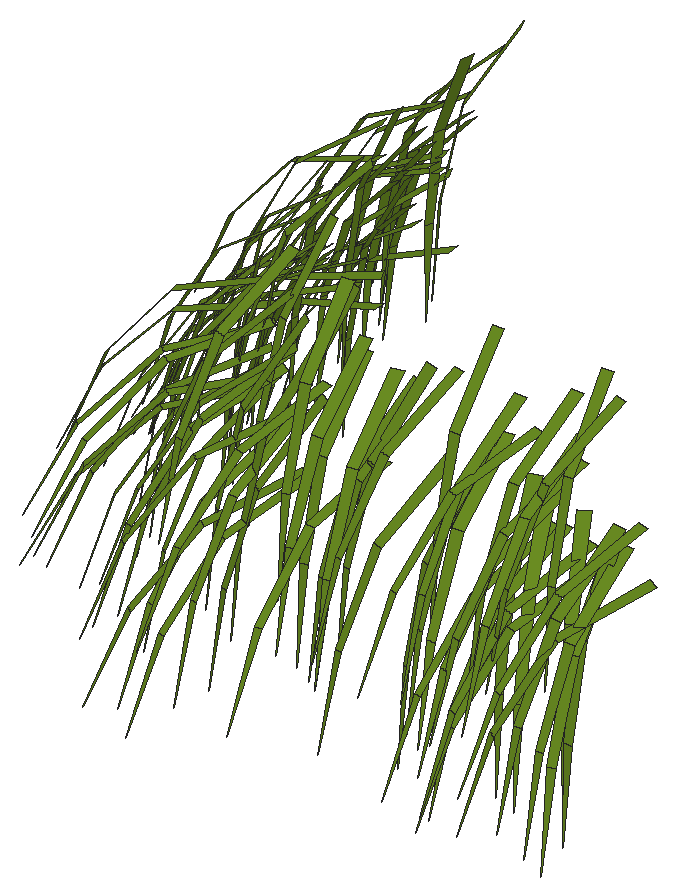
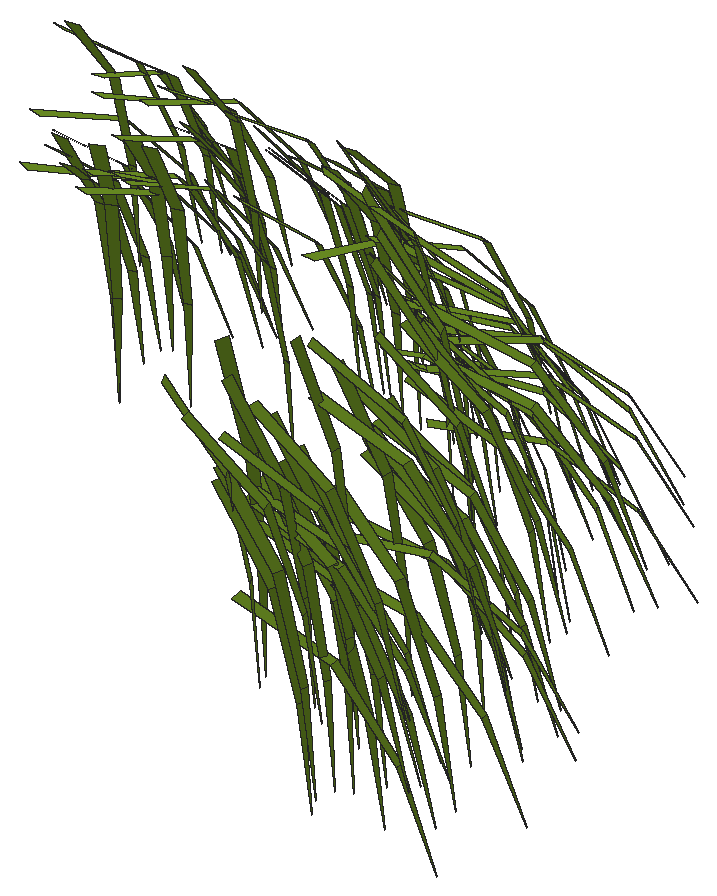
# SketchUp Ruby script. Lengths in inches.
U = 1.inch
M = Sketchup.active_model
def pt(a) = Geom::Point3d.new(a.map { |v| v * U })
def face(e, loops, mat)
  f = e.add_face(loops[0].map { |a| pt(a) })
  loops[1..].each { |l| e.add_face(l.map { |a| pt(a) }).erase! }
  f.material = f.back_material = mat if mat
  f
end
# faces: each face lists its corners as indices into pts; further lists are holes
def faces(e, pts, list, mat = nil) = list.each { |f| face(e, (f[0].is_a?(Array) ? f : [f]).map { |l| l.map { |i| pts[i] } }, mat) }
# xy, xz, yz: faces in a plane at the given z, y or x. An outline is a flat list of corners, or four numbers for a rectangle; further outlines are holes
def ring(l) = l.size == 4 ? [[l[0], l[1]], [l[2], l[1]], [l[2], l[3]], [l[0], l[3]]] : l.each_slice(2).to_a
def flat(e, list, mat, &to3) = list.each { |f| face(e, (f[0].is_a?(Array) ? f : [f]).map { |l| ring(l).map { |u, v| to3.(u, v) } }, mat) }
def xy(e, z, list, mat = nil) = flat(e, list, mat) { |x, y| [x, y, z] }
def xz(e, y, list, mat = nil) = flat(e, list, mat) { |x, z| [x, y, z] }
def yz(e, x, list, mat = nil) = flat(e, list, mat) { |y, z| [x, y, z] }
def lines(e, pts, list) = list.each { |a, b| e.add_line(pt(pts[a]), pt(pts[b])) }
# prism: a flat outline (further loops are holes) pulled along v
def prism(e, loops, v, mat = nil)
  f = face(e, loops, mat); d = Geom::Vector3d.new(v.map { |x| x * U })
  f.pushpull(f.normal.samedirection?(d) ? d.length : -d.length)
end
def box(e, o, s, mat = nil) = prism(e, [[o, [o[0] + s[0], o[1], o[2]], [o[0] + s[0], o[1] + s[1], o[2]], [o[0], o[1] + s[1], o[2]]]], [0, 0, s[2]], mat)
def at(x, y, z, deg = 0) = Geom::Transformation.translation(pt([x, y, z])) * Geom::Transformation.rotation(ORIGIN, Z_AXIS, deg.degrees)
def axes(o, x, y, z) = Geom::Transformation.new([*x, 0, *y, 0, *z, 0, *pt(o).to_a, 1])
def part(name) = M.definitions.add(name)
# library, detail: a bought-in or finely detailed component or shape, given as its bounding box
def library(name, o, s) = part(name).tap { |d| box(d.entities, o, s) }
def detail(e, o, s) = box(e.add_group.entities, o, s)
def put(e, d, t, mat = nil) = e.add_instance(d, t).tap { |i| i.material = mat if mat }
def group(e, t, mat = nil) = e.add_group.tap { |g| g.transformation = t; g.material = mat if mat }.entities
root = M.entities
M.materials.add("[0061_OliveDrab]").color = [107, 142, 35]
p = [[552.56,2.54,549.18],[552.375,2.61,549.18],[552.125,1.7,546.73],[563.22,4.1,549.35],[562.99,4.11,549.35],[563.1,3.94,546.73],
  [545.83,15.84,549.17],[545.8,16.0625,549.17],[544.89,15.83,546.72],[551.25,2.96,549.18],[551.09,3.08,549.18],[550.53,2.14,546.79],
  [563.64,2.99,549.4],[563.43,2.95,549.4],[563.65,2.43,546.84],[551.62,3.3,549.32],[551.44,3.35,549.32],[551.29,2.46,546.86],
  [563.01,4.3,549.51],[562.82,4.21,549.51],[562.99,4.09,546.89],[558.35,4.23,549.61],[558.15,4.32,549.61],[558.16,4.1,546.99],
  [547.34,11.93,549.62],[547.34,12.15,549.62],[546.97,12.05,547.02],[545.51,13.32,549.37],[545.49,13.53,549.37],[544.42,13.33,546.98],
  [563.41,2.8125,549.78],[563.2,2.82,549.78],[563.3,2.26,547.22],[550.85,4.72,549.82],[550.7,4.82,549.82],[550.51,4.39,547.23],
  [546.34,14.87,549.76],[546.33,15.08,549.76],[545.64,14.93,547.23],[546.98,15.4,549.77],[547.03,15.62,549.77],[546.49,15.62,547.2],
  [553.13,4.08,549.88],[552.95,4.19,549.88],[552.85,3.83,547.28],[561.19,4.14,549.96],[560.99,4.1,549.96],[561.13,3.95,547.34],
  [547.81,10.75,549.95],[547.78,10.98,549.95],[547.56,10.83,547.34],[546.36,13.86,549.79],[546.4,14.05,549.79],[545.74,14.11,547.25],
  [548.05,14.83,549.92],[548.05,15.02,549.92],[547.88,14.93,547.31],[553.04,3.125,549.95],[552.86,3.16,549.95],[552.84,2.5625,547.4],
  [548.61,5.67,550.06],[548.49,5.86,550.06],[547.88,5.34,547.56],[546.28,11.91,550.14],[546.28,12.12,550.14],[545.58,12.01,547.61],
  [561.52,1.93,550.16],[561.3,1.99,550.16],[561.14,1,547.73],[562.43,2.25,550.15],[562.23,2.35,550.15],[561.94,1.5,547.68],
  [557.39,2.96,550.26],[557.18,3.03,550.26],[557.12,2.48,547.69],[561.25,2.3,550.27],[561.06,2.32,550.27],[561.0625,1.58,547.76],
  [562.87,2.6875,550.3],[562.65,2.71,550.3],[562.68,2.03,547.76],[562.33,3.46,550.41],[562.13,3.37,550.41],[562.42,2.98,547.83],
  [545.73,11.7,550.1],[545.67,11.89,550.1],[544.57,11.45,547.75],[546.99,14.7,550.36],[546.89,14.9,550.36],[546.39,14.5,547.81],
  [547.1,10.29,550.52],[547.03,10.49,550.52],[546.6,10.22,547.95],[547.61,5.52,550.27],[547.49,5.66,550.27],[546.6,4.75,547.98],
  [546.375,11.93,550.44],[546.38,12.15,550.44],[545.55,12.07,547.95],[547.1,15.1,550.62],[547.15,15.27,550.62],[546.66,15.32,548.04],
  [561.51,1.99,550.54],[561.31,2.04,550.54],[561.19,1.11,548.09],[546.08,11.3,550.53],[546.05,11.5,550.53],[545.19,11.3,548.06],
  [560.51,1.94,550.64],[560.33,1.98,550.64],[560.2,0.95,548.23],[547.5,16.2,550.8],[547.55,16.38,550.8],[547.25,16.36,548.2],
  [550.9375,3.12,550.76],[550.77,3.25,550.76],[550.22,2.39,548.34],[545.82,11.72,550.62],[545.72,11.91,550.62],[544.66,11.24,548.31],
  [547.24,17.46,550.91],[547.27,17.66,550.91],[546.88,17.62,548.31],[548.42,5.11,550.85],[548.26,5.26,550.85],[547.625,4.45,548.43],
  [548.82,7.24,550.96],[548.68,7.39,550.96],[548.52,7.09,548.35],[546.26,10.83,550.88],[546.22,11.04,550.88],[545.52,10.8,548.36],
  [553.29,4.48,551.07],[553.09,4.58,551.07],[553.09,4.34,548.46],[556.15,1.63,551.02],[555.95,1.64,551.02],[555.99,0.57,548.62],
  [550.9,3.4,551.08],[550.71,3.5,551.08],[550.41,2.65,548.62],[559.3125,3.52,551.24],[559.13,3.55,551.24],[559.16,3.17,548.65],
  [547.9375,8.1,551.17],[547.83,8.26,551.17],[547.53,7.95,548.58],[546.76,8.87,551.09],[546.7,9.04,551.09],[545.92,8.65,548.62],
  [551.09,3.81,551.23],[550.91,3.93,551.23],[550.61,3.31,548.69],[552.31,4.83,551.36],[552.16,4.93,551.36],[552.09,4.68,548.75],
  [547.66,9.04,551.28],[547.63,9.24,551.28],[547.2,9.07,548.69],[547.14,17.42,551.29],[547.18,17.62,551.29],[546.79,17.59,548.69],
  [548.11,12.78,551.42],[548.12,12.99,551.42],[547.9375,12.89,548.8],[547.6,15.3,551.43],[547.62,15.52,551.43],[547.33,15.4375,548.82],
  [556.73,3.44,551.49],[556.53,3.49,551.49],[556.54,3.09,548.9],[555.7,3.87,551.55],[555.49,3.86,551.55],[555.6,3.61,548.94],
  [546.04,16.18,551.39],[546.07,16.39,551.39],[545.21,16.4,548.91],[556.43,3.54,551.58],[556.22,3.61,551.58],[556.22,3.25,548.97],
  [561.23,1.99,551.57],[561.09,2,551.57],[561.11,1.125,549.09],[561.29,1.99,551.57],[560.32,2.74,551.65],[560.11,2.71,551.65],
  [560.28,2.15,549.09],[550.51,4.14,551.55],[550.37,4.3,551.55],[549.79,3.66,549.07],[546.1,15.28,551.58],[546.06,15.46,551.58],
  [545.3,15.19,549.08],[545.67,15.77,551.53],[545.65,15.96,551.53],[544.56,15.79,549.15],[562.91,1.875,551.58],[562.72,1.92,551.58],
  [562.54,0.81,549.2],[553.18,4.01,551.26],[552.92,4.12,551.26],[552.29,4.33,551.16],[552.07,4.5,551.16],[556.88,3.91,551.83],
  [556.67,3.98,551.83],[556.69,3.68,549.22],[547.68,10.27,551.81],[547.62,10.44,551.81],[547.32,10.23,549.21],[547.44,16.02,551.23],
  [547.4,16.33,551.23],[552.0625,4.75,551.47],[551.81,4.82,551.47],[548.98,4.11,551.66],[548.83,4.27,551.66],[548.05,3.42,549.3],
  [563.27,4.59,551.93],[562.95,4.59,551.93],[546.56,12.1,551.84],[546.54,12.29,551.84],[545.94,12.14,549.28],[563.46,4.0625,551.79],
  [563.17,4,551.79],[550.47,4.96,552.02],[550.32,5.11,552.02],[550.05,4.68,549.44],[547.31,13.43,551.28],[547.28,13.73,551.28],
  [553.29,2.2,551.86],[553.1,2.25,551.86],[552.87,1.16,549.48],[557.15,2.92,552.05],[556.94,2.89,552.05],[557.13,2.34,549.49],
  [562.83,4.78,552.09],[562.57,4.66,552.09],[546.58,7.67,551.83],[546.53,7.88,551.83],[545.49,7.49,549.45],[558.61,4.67,552.18],
  [558.32,4.81,552.18],[547.86,5.29,551.86],[547.73,5.41,551.86],[546.96,4.41,549.56],[548.14,11.875,552.12],[548.15,12.18,552.12],
  [548.9,13.7,552.17],[548.89,13.9,552.17],[548.76,13.79,549.55],[546.8,9.9,552.21],[546.8,10.09,552.21],[546.02,9.96,549.7],
  [561.45,2.19,552.34],[561.24,2.23,552.34],[561.2,1.44,549.83],[555.89,3.12,552.37],[555.68,3.1,552.37],[555.83,2.53,549.8125],
  [563.47,3.92,552.16],[563.17,3.92,552.16],[551.43,5.49,552.26],[551.22,5.64,552.26],[554.12,5.14,552.4],[553.93,5.22,552.4],
  [553.96,5.04,549.78],[547.61,13.52,552.08],[547.67,13.78,552.08],[547.65,14.91,552.04],[547.63,15.2,552.04],[547.97,15.15,552.19],
  [548.04,15.45,552.19],[548.87,4.33,552.18],[548.68,4.44,552.18],[548.11,3.28,549.9],[553.58,4.74,552.38],[553.33,4.89,552.38],
  [548.53,14.79,552.5],[548.53,15.0625,552.5],[548.19,16.08,552.55],[548.19,16.28,552.55],[547.96,16.18,549.93],[553.3,4.27,552.3],
  [553.04,4.32,552.3],[561.13,4.64,552.53],[560.83,4.57,552.53],[548.43,10.79,552.5],[548.39,11.11,552.5],[546.66,15.59,552.53],
  [546.6,15.77,552.53],[545.9375,15.45,550.01],[563.17,3.66,552.23],[562.89,3.8,552.23],[549.8,6.36,552.29],[549.63,6.625,552.29],
  [546.98,7.35,552.51],[546.93,7.5625,552.51],[546.03,7.21,550.07],[549.66,8.78,552.75],[549.58,8.97,552.75],[549.45,8.8,550.14],
  [548.9,9.77,552.71],[548.84,9.94,552.71],[548.66,9.79,550.09],[547.49,12.2,551.98],[547.4,12.47,551.98],[547.6,11.89,552.41],
  [547.6,12.18,552.41],[562.02,3.53,552.17],[561.71,3.62,552.17],[549.375,16.06,552.86],[549.43,16.28,552.86],[549.28,16.2,550.24],
  [547.54,16.96,552.77],[547.48,17.17,552.77],[547.125,16.96,550.17],[560.1,2.66,552.82],[559.9,2.66,552.82],[559.99,1.91,550.3],
  [557.57,2.74,552.84],[557.38,2.79,552.84],[557.31,2.02,550.33],[561.47,3.66,552.51],[561.1875,3.7,552.51],[563.06,3.9,552.62],
  [562.75,3.9375,552.62],[557.75,3.98,552.65],[557.45,4.08,552.65],[549.1,6.78,552.03],[548.92,6.98,552.03],[561.99,4.35,552.86],
  [561.71,4.23,552.86],[554.97,4.13,553.02],[554.77,4.1,553.02],[554.93,3.74,550.42],[552.45,6.26,553.05],[552.27,6.3125,553.05],
  [552.27,6.01,550.4375],[547.74,11.85,552.6875],[547.75,12.16,552.6875],[548.07,15.25,552.69],[547.91,15.52,552.69],[549.15,16.86,552.99],
  [549.04,17.05,552.99],[548.93,16.86,550.375],[561.92,3.55,552.61],[561.64,3.62,552.61],[561.42,3.2,553.12],[561.21,3.21,553.12],
  [561.28,2.72,550.54],[559.11,4.43,553.09],[558.92,4.43,553.09],[559.02,4.16,550.48],[562.44,4.46,553.07],[562.25,4.45,553.07],
  [562.37,4.17,550.46],[550.76,8.13,553.14],[550.66,8.34,553.14],[550.5625,8.16,550.52],[548.09,10.61,552.93],[547.99,10.88,552.93],
  [547.57,11.42,552.6875],[547.53,11.71,552.6875],[546.32,15.93,553.01],[546.34,16.13,553.01],[545.56,16.1,550.51],[562.4,2.11,553.05],
  [562.21,2.09,553.05],[562.4,1.11,550.625],[560.91,3.57,552.66],[560.65,3.625,552.66],[551.57,4.43,553.13],[551.37,4.47,553.13],
  [551.34,3.87,550.58],[547.6,12.59,552.34],[547.46,12.86,552.34],[547.03,12.43,553.15],[546.97,12.62,553.15],[546.44,12.34,550.6],
  [545.75,13.43,553.01],[545.74,13.66,553.01],[544.7,13.5,550.61],[548.02,14.79,553.05],[548.09,15.04,553.05],[559.79,1.96,553.09],
  [559.61,2,553.09],[559.46,1,550.67],[561.94,3.38,553.29],[561.74,3.4375,553.29],[561.6875,2.9,550.72],[552.01,4.41,552.77],
  [551.79,4.59,552.77],[548.18,15.98,553.33],[548.24,16.23,553.33],[549.63,6.28,552.86],[549.41,6.5,552.86],[547.63,11.05,553.11],
  [547.57,11.35,553.11],[548.06,17.3,553.39],[548.1,17.58,553.39],[556.29,3.41,552.95],[556.01,3.42,552.95],[549.41,7.76,553.46],
  [549.22,7.96,553.46],[551.63,4.78,553.2],[551.36,4.92,553.2],[553.59,4.97,553.64],[553.3125,5.11,553.64],[548.125,9.35,553.29],
  [548.03,9.59,553.29],[559.48,4.33,553.74],[559.23,4.37,553.74],[551.85,4.84,553.52],[551.6,5.01,553.52],[553.74,6.27,552.18],
  [553.46,6.47,552.18],[548.74,8.59,553.625],[548.59,8.82,553.625],[549.86,16.32,552.2],[549.8125,16.7,552.2],[554.09,6.25,552.3],
  [553.78,6.37,552.3],[548.59,9.14,553.73],[548.55,9.42,553.73],[549.85,13.61,551.89],[549.82,13.98,551.89],[547.99,17.21,553.77],
  [548.04,17.5,553.77],[552.69,5.31,553.91],[552.48,5.46,553.91],[548.61,12.72,554],[548.62,13.02,554],[548.29,15.18,553.96],
  [548.32,15.49,553.96],[547.51,15.93,553.55],[547.55,16.23,553.55],[556.97,4.27,553.97],[556.7,4.34,553.97],[552.7,6.96,552.73],
  [552.39,7.05,552.73],[547.41,15.84,553.49],[547.39,16.11,553.49],[563.37,3.5625,553.54],[563.1,3.63,553.54],[561.47,3.53,553.68],
  [561.18,3.56,553.68],[556.74,4.3,554.07],[556.44,4.4,554.07],[555.73,4.54,554.09],[555.43,4.53,554.09],[551.63,5.03,553.75],
  [551.43,5.26,553.75],[547.54,15.57,553.75],[547.48,15.83,553.75],[560.24,3.89,554.01],[559.93,3.86,554.01],[550.41,5.36,553.47],
  [550.2,5.59,553.47],[557.14,4.55,554.37],[556.83,4.65,554.37],[563.1,6,553.53],[562.74,5.92,553.53],[550.93,7.55,554.375],
  [550.78,7.71,554.375],[550.57,7.34,551.78],[548.34,8.08,553.74],[548.26,8.39,553.74],[548.48,10.53,554.29],[548.38,10.78,554.29],
  [547.76,12.17,554.17],[547.73,12.45,554.17],[553.82,3.85,553.82],[553.5625,3.93,553.82],[563.33,5.96,554.17],[562.94,5.96,554.17],
  [549.2,6.74,553.59],[549,6.92,553.59],[551.23,5.6875,554.42],[551.02,5.89,554.42],[551.05,8.46,552.5625],[550.83,8.71,552.5625],
  [549.89,12.91,552.77],[549.79,13.24,552.77],[549.85,15,553.47],[549.83,15.36,553.47],[557.02,4.05,554.42],[556.73,4,554.42],
  [562.27,6.04,554.32],[561.95,5.88,554.32],[549.83,11.8125,554.125],[549.84,12.18,554.125],[549.8,12.95,553.41],[549.875,13.28,553.41],
  [562.72,5.91,553.05],[562.34,6.01,553.05],[564.28,5.875,553.1],[563.94,6.04,553.1],[563.54,5.96,553.82],[563.17,5.96,553.82],
  [549.93,6.01,553.91],[549.67,6.16,553.91],[559.21,5.88,554.4375],[558.86,6.04,554.4375],[548.16,9.92,554.46],[548.15,10.1875,554.46],
  [549.28,13.68,554.77],[549.26,13.97,554.77],[549.8,14.73,554.03],[549.875,15.1,554.03],[561.75,3.62,554.52],[561.46,3.68,554.52],
  [553.73,6.35,553.84],[553.4,6.41,553.84],[552.52,7.02,554.09],[552.26,7.2,554.09],[551.67,7.49,553.74],[551.47,7.82,553.74],
  [549.92,13.76,552.68],[549.75,14.09,552.68],[555.83,4.25,554.74],[555.53,4.22,554.74],[554.47,6.14,554.42],[554.16,6.32,554.42],
  [554.35,5.53,554.99],[554.09,5.65,554.99],[549.84,11.89,553.78],[549.83,12.25,553.78],[561.79,5.9375,553.77],[561.44,5.98,553.77],
  [560.85,6,554.76],[560.49,5.92,554.76],[548.61,7.74,554.54],[548.53,8.04,554.54],[549.99,10.97,554.6],[549.9375,11.36,554.6],
  [549.84,14.75,554.78],[549.84,15.08,554.78],[547.9375,15.97,554.79],[547.85,16.23,554.79],[548.8,16.04,555.1],[548.8,16.33,555.1],
  [562.53,5.92,553.57],[562.18,6,553.57],[563.33,5.9375,554.25],[562.96,5.98,554.25],[561.45,5.93,553.68],[561.14,5.99,553.68],
  [558.39,5.9,554.33],[558.02,6.02,554.33],[549.47,9.92,555.27],[549.38,10.17,555.27],[549.86,11.65,553.95],[549.82,12,553.95],
  [549.83,11.75,554.27],[549.84,12.13,554.27],[549.93,16.24,554.25],[549.74,16.57,554.25],[557.91,4.05,555.09],[557.64,4.11,555.09],
  [560.17,3.99,555.08],[559.89,4,555.08],[553.5625,6.31,553.72],[553.28,6.53,553.72],[550.17,8.94,555.32],[550.06,9.22,555.32],
  [548.42,17.15,555.23],[548.34,17.44,555.23],[556.48,5.95,553.58],[556.13,5.97,553.58],[561.3,6.03,554.76],[560.96,5.89,554.76],
  [551.37,8.01,553.81],[551.1,8.28,553.81],[549.97,11.27,554.64],[549.85,11.61,554.64],[549.73,15.93,555.46],[549.8,16.24,555.46],
  [549.61,15.97,554.62],[554.89,5,555.49],[554.61,4.96,555.49],[552.68,6.86,555.59],[552.43,6.9375,555.59],[547.47,13.46,555],
  [547.46,13.77,555],[547.74,15.75,555.22],[547.76,16.04,555.22],[549.62,17.08,555.57],[549.47,17.34,555.57],[560.24,3.61,555.08],
  [559.98,3.67,555.08],[562.29,3.74,555.1],[562.02,3.72,555.1],[561.55,4.25,555.52],[561.25,4.27,555.52],[551.88,5.58,555.47],
  [551.59,5.65,555.47],[559.13,5.12,555.63],[558.86,5.11,555.63],[562.42,5.16,555.6],[562.15,5.14,555.6],[551.21,8.29,555.72],
  [551.07,8.58,555.72],[549.91,11.45,554.35],[549.83,11.83,554.35],[549.79,14.25,554.91],[549.88,14.55,554.91],[552.72,6.92,554.26],
  [552.38,7.08,554.26],[548.18,12.75,555.49],[548.09,13.02,555.49],[562.29,4.43,555.67],[562.02,4.51,555.67],[562.24,4.28,555.34],
  [550.2,10.12,554.7],[550.09,10.41,554.7],[549.8,15.52,555.34],[549.88,15.83,555.34],[549.8125,17,555.32],[549.86,17.34,555.32],
  [563.99,5.92,554.51],[563.65,6,554.51],[553.12,6.62,554.97],[552.81,6.83,554.97],[552.35,7.08,553.87],[552.1,7.36,553.87],
  [550.73,8.98,555.375],[550.49,9.23,555.375],[549.85,15.96,554.45],[549.83,16.3,554.45],[554.31,6.29,555.79],[553.96,6.46,555.79],
  [550.93,8.66,554.03],[550.7,8.875,554.03],[550.36,9.63,555.41],[550.17,9.91,555.41],[549.8125,15.57,554.75],[549.86,15.9375,554.75],
  [561.72,5.94,554.69],[561.37,5.98,554.69],[559.8,6.01,555.72],[559.48,6.0625,555.72],[550.79,8.7,554.45],[550.69,9.07,554.45],
  [550.41,9.38,555.61],[550.36,9.73,555.61],[549.875,16.08,554.84],[549.8,16.39,554.84],[554.55,6.17,554.82],[554.23,6.26,554.82],
  [553.32,6.43,555.2],[553.08,6.71,555.2],[549.85,16.82,555.57],[549.92,17.17,555.57],[553.6,6.53,556.05],[553.34,6.72,556.05],
  [551.29,8.2,554.37],[550.97,8.39,554.37],[560.04,6.02,555.53],[559.67,5.98,555.53],[557.43,6.03,555.87],[557.1,6.11,555.87],
  [550.01,12.65,556.22],[550.02,13.02,556.22],[549.95,14.97,555.98],[549.99,15.35,555.98],[557.35,6.02,555.95],[556.99,6.14,555.95],
  [555.74,6.18,556.14],[555.37,6.17,556.14],[549.92,12.35,555.65],[549.89,12.6875,555.65],[550.2,11.15,556.18],[550.08,11.45,556.18],
  [556.73,6.12,556],[556.38,6.07,556],[557.67,6.11,556.4],[557.3,6.23,556.4],[552.67,7.13,556.08],[552.42,7.38,556.08],
  [551.63,8.18,556.83],[551.41,8.39,556.83],[562.22,5.98,555.58],[561.86,6.04,555.58],[551.03,8.35,555.35],[550.93,8.71,555.35],
  [550.32,9.99,555.94],[550.31,10.3125,555.94],[555.68,6.27,556.41],[555.32,6.24,556.41],[550.33,13.71,557.17],[550.31,14.07,557.17],
  [550.06,16.64,556.18],[549.95,16.96,556.18],[554.9375,6.71,557.26],[554.625,6.86,557.26],[549.95,13.52,555.86],[549.94,13.91,555.86],
  [560.86,6.03,555.88],[560.55,6.11,555.88],[562.09,6.14,556.15],[561.77,6.11,556.15],[558.42,6.17,556.55],[558.09,6.24,556.55],
  [560.24,6.19,556.51],[559.89,6.2,556.51],[550.35,16.02,557.22],[550.35,16.37,557.22],[550.04,15.51,556.45],[550.08,15.86,556.45],
  [550.27,17.6,557.03],[550.18,17.96,557.03],[551.5,9.47,557.52],[551.36,9.81,557.52],[550.91,10.37,557.41],[550.81,10.68,557.41],
  [561.76,6.36,557.07],[561.39,6.39,557.07],[554.65,6.9,557.29],[554.3,6.85,557.29],[552.39,7.71,556.92],[552.05,7.79,556.92],
  [550.25,13.37,556.98],[550.14,13.7,556.98],[550.74,15.64,557.87],[550.83,16.02,557.87],[559.11,6.77,557.66],[558.79,6.76,557.66],
  [562.32,6.78,557.66],[561.98,6.75,557.66],[553.14,8.18,557.8125],[552.84,8.28,557.8125],[550.83,17.73,557.8],[550.65,18.06,557.8],
  [562.92,6.4375,557.24],[562.59,6.54,557.24],[552.43,8.84,557.98],[552.26,9.19,557.98],[552.13,9.125,557.72],[553.06,9.55,558.55],
  [552.8,9.81,558.55]]
faces(root,p,[[0,1,2],[3,4,5],[6,7,8],[9,10,11],[12,13,14],[15,16,17],[18,19,20],[21,22,23],
  [24,25,26],[27,28,29],[30,31,32],[33,34,35],[36,37,38],[39,40,41],[42,43,44],[45,46,47],
  [48,49,50],[51,52,53],[54,55,56],[57,58,59],[60,61,62],[63,64,65],[66,67,68],[69,70,71],
  [72,73,74],[75,76,77],[78,79,80],[81,82,83],[84,85,86],[87,88,89],[90,91,92],[93,94,95],
  [96,97,98],[99,100,101],[102,103,104],[105,106,107],[108,109,110],[111,112,113],[114,115,116],[117,118,119],
  [120,121,122],[123,124,125],[126,127,128],[129,130,131],[132,133,134],[135,136,137],[138,139,140],[141,142,143],
  [144,145,146],[147,148,149],[150,151,152],[153,154,155],[156,157,158],[159,160,161],[162,163,164],[165,166,167],
  [168,169,170],[171,172,173],[174,175,176],[177,178,179],[180,181,182,183],[184,185,186],[187,188,189],[190,191,192],
  [193,194,195],[196,197,198],[199,200,1,0],[201,202,10,9],[203,204,205],[206,207,208],[209,210,7,6],[211,212,16,15],
  [213,214,215],[216,217,4,3],[218,219,220],[221,222,13,12],[223,224,225],[226,227,28,27],[228,229,230],[231,232,233],
  [234,235,19,18],[236,237,238],[239,240,22,21],[241,242,243],[244,245,25,24],[246,247,248],[249,250,251],[252,253,180,254],
  [255,256,257],[258,259,31,30],[260,261,34,33],[262,263,264],[265,266,52,51],[267,268,37,36],[269,270,40,39],[271,272,273],
  [274,275,43,42],[276,277,55,54],[278,279,280],[281,282,58,57],[283,284,46,45],[285,286,49,48],[287,288,289],[290,291,70,69],
  [292,293,61,60],[294,295,296],[297,298,299],[300,301,302],[303,304,85,84],[305,306,64,63],[307,308,67,66],[309,310,311],
  [312,313,314],[315,316,317],[318,319,320],[321,322,76,75],[323,324,79,78],[325,326,73,72],[327,328,94,93],[329,330,82,81],
  [331,332,333],[334,335,336],[337,338,97,96],[339,340,88,87],[341,342,343],[344,345,103,102],[346,347,348],[349,350,351],
  [352,353,354],[355,356,357],[358,359,91,90],[360,361,106,105],[362,363,364],[365,366,367],[368,369,109,108],[370,371,372],
  [373,374,118,117],[375,376,377],[378,379,380],[381,382,100,99],[383,384,385],[386,387,388],[389,390,115,114],[391,392,112,111],
  [393,394,124,123],[395,396,130,129],[397,398,121,120],[399,400,136,135],[401,402,127,126],[403,404,139,138],[405,406,133,132],[407,408,148,147],
  [409,410,142,141],[411,412,151,150],[413,414,202,201],[415,416,145,144],[417,418,210,209],[419,420,200,199],[421,422,157,156],[423,424,227,226],
  [425,426,160,159],[427,428,154,153],[429,430,163,162],[431,432,166,165],[433,434,175,174],[435,436,169,168],[437,438,212,211],[439,440,194,193],
  [441,442,197,196],[443,444,181,180,183],[445,446,178,177],[447,448,172,171],[449,450,188,187],[451,452,191,190],[453,454,185,184],[455,456,214,213],
  [457,458,204,203],[459,460,222,221],[461,462,463],[464,465,237,236],[466,467,207,206],[468,469,219,218],[470,471,229,228],[472,473,217,216],
  [474,475,242,241],[476,477,224,223],[478,479,328,327],[480,481,304,303],[482,483,268,267],[484,485,232,231],[486,487,235,234],[488,489,245,244],
  [490,491,266,265],[492,493,308,307],[494,495,291,290],[496,497,259,258],[498,499,272,271],[500,501,240,239],[502,503,250,249],[504,505,247,246],
  [506,507,270,269],[508,509,253,252],[510,511,282,281],[512,513,261,260],[514,515,293,292],[516,517,374,373],[518,519,256,255],[520,521,275,274],
  [522,523,263,262],[524,525,306,305],[526,527,322,321],[528,529,284,283],[530,531,295,294],[532,533,286,285],[534,535,277,276],[536,537,288,287],
  [538,539,279,278],[540,541,345,344],[542,543,324,323],[544,545,369,368],[546,547,326,325],[548,549,301,300],[550,551,361,360],[552,553,338,337],
  [554,555,340,339],[556,557,319,318],[558,559,316,315],[560,561,390,389],[562,563,298,297],[564,565,313,312],[566,567,400,399],[568,569,330,329],
  [570,571,394,393],[572,573,359,358],[574,575,310,309,576],[577,578,332,331],[579,580,335,334],[581,582,379,378],[583,584,363,362],[585,586,342,341],
  [587,588,384,383],[589,590,366,365],[591,592,347,346],[593,594,371,370],[595,596,350,349],[597,598,353,352],[599,600,356,355],[601,602,396,395],
  [603,604,382,381],[605,606,404,403],[607,608,376,375],[609,610,387,386,611],[612,613,408,407],[614,615,392,391],[616,617,398,397],[618,619,442,441],
  [620,621,412,411],[622,623,456,455],[624,625,402,401],[626,627,440,439],[628,629,406,405],[630,631,475,474],[632,633,416,415],[634,635,576,434,433],
  [636,637,444,443],[638,639,410,409],[640,641,465,464],[642,643,422,421],[644,645,452,451],[646,647,471,470],[648,649,450,449],[650,651,426,425],
  [652,653,428,427],[654,655,499,498],[656,657,454,453],[658,659,436,435],[660,661,430,429],[662,663,432,431],[664,665,446,445],[666,667,448,447],
  [668,669,469,468],[670,671,467,466],[672,673,485,484],[674,675,458,457],[676,677,477,476],[678,679,462,461],[680,681,509,508],[682,683,531,530],
  [684,685,503,502],[686,687,519,518],[688,689,505,504],[690,691,537,536],[692,693,523,522],[694,695,582,581],[696,697,588,587],[698,699,590,589,611],
  [700,701,557,556],[702,703,559,558],[704,705,539,538],[706,707,584,583],[708,709,565,564],[710,711,563,562],[712,713,549,548],[714,715,592,591],
  [716,717,578,577],[718,719,594,593],[720,721,608,607],[722,723,575,574],[724,725,596,595],[726,727,598,597],[728,729,580,579],[730,731,586,585],
  [732,733,610,609],[734,735,736,600,599],[737,738,736,679,678]],"[0061_OliveDrab]")
